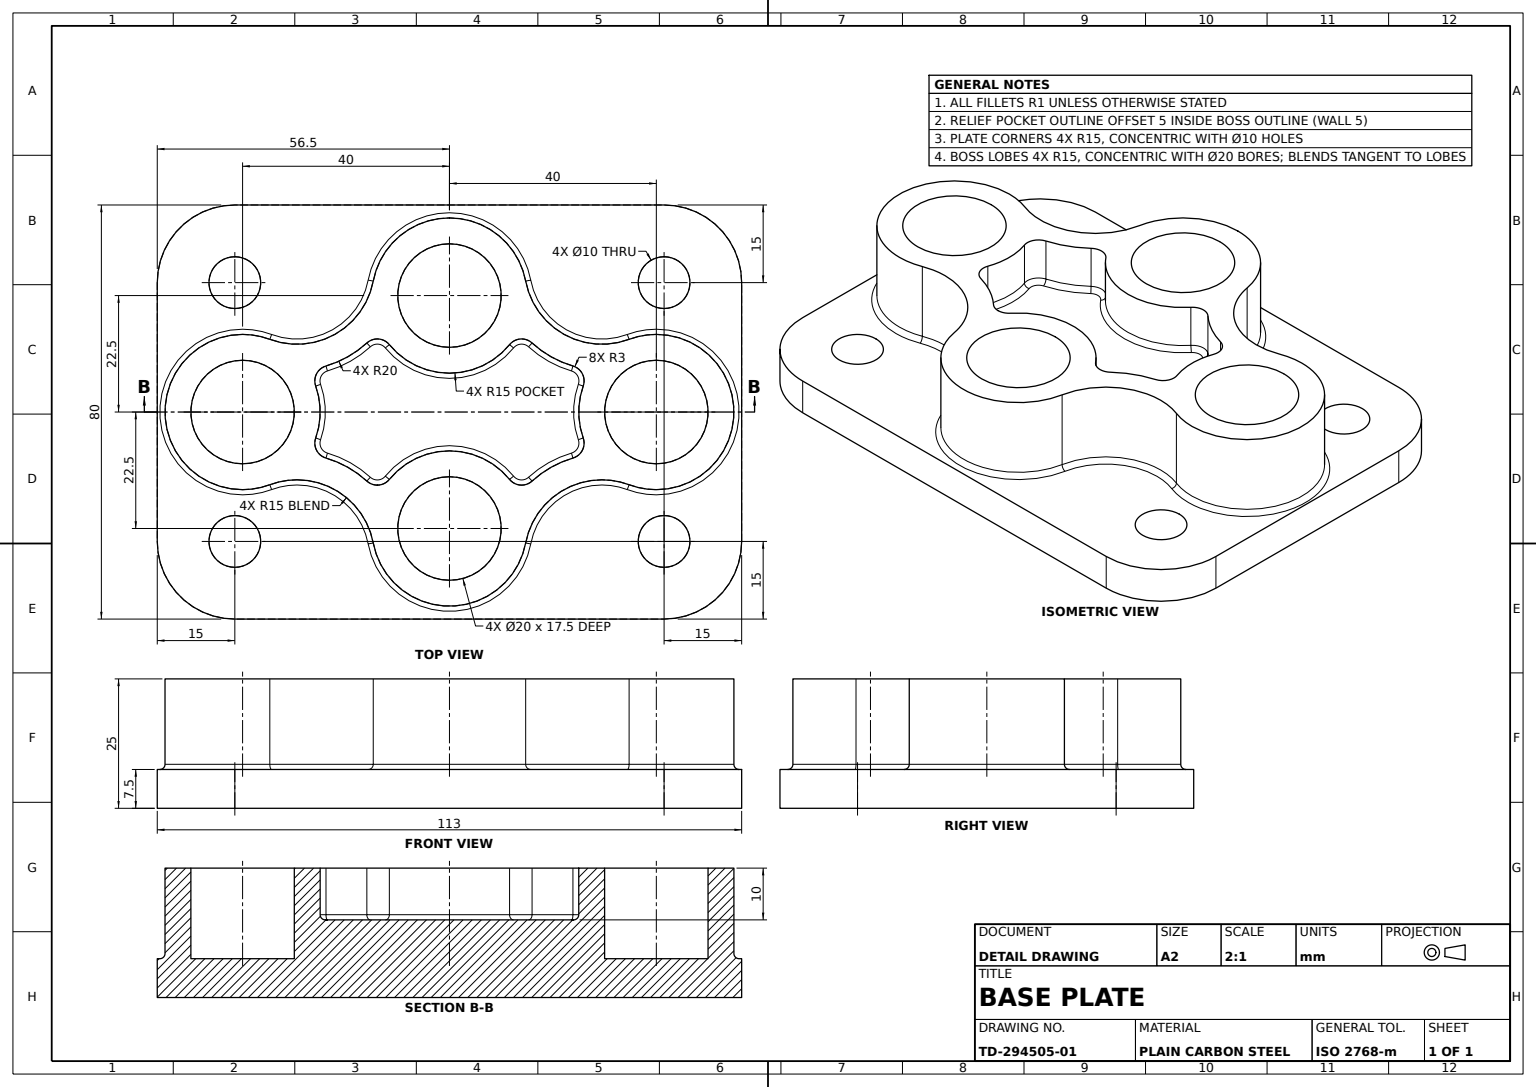
solid
v1 (-56.5,0,25)
v2 (-56.5,7.5,25)
e1 v1 v2 LINE
v3 (-41.5,0,40)
e2 v3 v1 CIRCLE(AX(P(-41.5,0,25),D(0,-1,0),D(0,0,-1)),15)
v4 (-41.5,7.5,40)
e3 v4 v3 LINE
e4 v2 v4 CIRCLE(AX(P(-41.5,7.5,25),D(0,1,0),D(0,0,-1)),15)
face CYL(AX(P(-41.5,7.5,25),D(0,-1,0),D(0,0,-1)),15) [-e1 -e2 -e3 -e4]
v5 (41.5,7.5,20)
v6 (41.5,7.5,30)
e5 v5 v6 CIRCLE(AX(P(41.5,7.5,25),D(0,1,0),D(0,0,1)),5)
v7 (41.5,0,30)
e6 v7 v6 LINE
v8 (41.5,0,20)
e7 v8 v7 CIRCLE(AX(P(41.5,0,25),D(0,1,0),D(0,0,1)),5)
e8 v8 v5 LINE
face CYL(AX(P(41.5,0,25),D(0,1,0),D(0,0,1)),5) rev [e5 -e6 -e7 e8]
v9 (0,7.5,-12.5)
v10 (0,7.5,-32.5)
e9 v9 v10 CIRCLE(AX(P(0,7.5,-22.5),D(0,1,0),D(0,0,1)),10)
e10 v10 v9 CIRCLE(AX(P(0,7.5,-22.5),D(0,1,0),D(0,0,1)),10)
face PLANE(AX(P(0,7.5,0),D(0,-1,0),D(0,0,-1))) rev [e9 e10]
v11 (25.861645,16,5.01068)
v12 (25.861645,25,5.01068)
e11 v11 v12 LINE
v13 (25.861645,25,-5.01068)
e12 v12 v13 CIRCLE(AX(P(40,25,0),D(0,-1,0),D(0,0,1)),15)
v14 (25.861645,16,-5.01068)
e13 v14 v13 LINE
e14 v14 v11 CIRCLE(AX(P(40,16,0),D(0,1,0),D(0,0,1)),15)
face CYL(AX(P(40,15,0),D(0,1,0),D(0,0,1)),15) [e11 e12 -e13 e14]
v15 (40,7.5,-16)
v16 (40,8.5,-15)
e15 v15 v16 CIRCLE(AX(P(40,8.5,-16),D(-1,0,0),D(0,0,1)),1)
v17 (34.38617,7.5,-14.982821)
e16 v17 v15 CIRCLE(AX(P(40,7.5,0),D(0,-1,0),D(0,0,-1)),16)
v18 (34.737034,8.5,-14.046394)
e17 v17 v18 CIRCLE(AX(P(34.38617,8.5,-14.982821),D(-0.936426284,0,0.350864382),D(0.350864382,0,0.936426284)),1)
e18 v16 v18 CIRCLE(AX(P(40,8.5,0),D(0,1,0),D(0,0,-1)),15)
face TORUS(AX(P(40,8.5,0),D(0,-1,0),D(0,0,-1)),16,1) rev [-e15 -e16 e17 -e18]
v19 (40,25,-15)
e19 v19 v16 LINE
v20 (40,25,15)
e20 v20 v19 CIRCLE(AX(P(40,25,0),D(0,1,0),D(0,0,1)),15)
v21 (40,8.5,15)
e21 v20 v21 LINE
e22 v21 v16 CIRCLE(AX(P(40,8.5,0),D(0,1,0),D(0,0,-1)),15)
face CYL(AX(P(40,25,0),D(0,-1,0),D(0,0,-1)),15) [-e19 -e20 e21 e22]
v22 (-12.398933,15,12.387312)
v23 (12.398933,15,12.387312)
e23 v22 v23 CIRCLE(AX(P(0,15,22.5),D(0,-1,0),D(0,0,1)),16)
v24 (-11.624,16,13.019355)
e24 v22 v24 CIRCLE(AX(P(-12.398933,16,12.387312),D(-0.632042977,0,0.774933336),D(0.774933336,0,0.632042977)),1)
v25 (11.624,16,13.019355)
e25 v25 v24 CIRCLE(AX(P(0,16,22.5),D(0,1,0),D(0,0,1)),15)
e26 v23 v25 CIRCLE(AX(P(12.398933,16,12.387312),D(-0.632042977,0,-0.774933336),D(-0.774933336,0,0.632042977)),1)
face TORUS(AX(P(0,16,22.5),D(0,1,0),D(0,0,1)),16,1) rev [-e23 e24 -e25 -e26]
v26 (40,7.5,16)
e27 v26 v21 CIRCLE(AX(P(40,8.5,16),D(1,0,0),D(0,0,-1)),1)
e28 v15 v26 CIRCLE(AX(P(40,7.5,0),D(0,-1,0),D(0,0,-1)),16)
face TORUS(AX(P(40,8.5,0),D(0,-1,0),D(0,0,-1)),16,1) rev [e15 -e22 -e27 -e28]
v27 (-56.5,7.5,-25)
e29 v27 v2 LINE
v28 (-56.5,0,-25)
e30 v27 v28 LINE
e31 v28 v1 LINE
face PLANE(AX(P(-56.5,7.5,40),D(1,0,0),D(0,0,-1))) rev [e1 -e29 e30 e31]
v29 (-13.9488,15,13.123226)
v30 (-13.9488,16,14.123226)
e32 v29 v30 CIRCLE(AX(P(-13.9488,16,13.123226),D(-1,0,0),D(0,0,1)),1)
v31 (-15.298823,15,12.598841)
e33 v31 v29 CIRCLE(AX(P(-13.9488,15,11.123226),D(0,1,0),D(0,0,1)),2)
v32 (-15.973835,16,13.336648)
e34 v32 v31 CIRCLE(AX(P(-15.298823,16,12.598841),D(0.737807048,0,0.675011674),D(0.675011674,0,-0.737807048)),1)
e35 v30 v32 CIRCLE(AX(P(-13.9488,16,11.123226),D(0,-1,0),D(0,0,1)),3)
face TORUS(AX(P(-13.9488,16,11.123226),D(0,1,0),D(0,0,1)),2,1) rev [-e32 -e33 -e34 -e35]
v33 (34.737034,25,-14.046394)
e36 v33 v18 LINE
e37 v19 v33 CIRCLE(AX(P(40,25,0),D(0,1,0),D(0,0,1)),15)
face CYL(AX(P(40,25,0),D(0,-1,0),D(0,0,-1)),15) [-e36 -e37 e19 e18]
v34 (0,25,-32.5)
e38 v34 v10 LINE
v35 (0,25,-12.5)
e39 v34 v35 CIRCLE(AX(P(0,25,-22.5),D(0,1,0),D(0,0,1)),10)
e40 v35 v9 LINE
face CYL(AX(P(0,25,-22.5),D(0,-1,0),D(0,0,-1)),10) rev [-e38 e39 e40 -e10]
v36 (-34.737034,8.5,-14.046394)
v37 (-40,8.5,-15)
e41 v36 v37 CIRCLE(AX(P(-40,8.5,0),D(0,1,0),D(0,0,-1)),15)
v38 (-34.38617,7.5,-14.982821)
e42 v36 v38 CIRCLE(AX(P(-34.38617,8.5,-14.982821),D(0.936426284,0,0.350864382),D(0.350864382,0,-0.936426284)),1)
v39 (-40,7.5,-16)
e43 v39 v38 CIRCLE(AX(P(-40,7.5,0),D(0,-1,0),D(0,0,-1)),16)
e44 v39 v37 CIRCLE(AX(P(-40,8.5,-16),D(-1,0,0),D(0,0,1)),1)
face TORUS(AX(P(-40,8.5,0),D(0,-1,0),D(0,0,-1)),16,1) rev [-e41 e42 -e43 e44]
v40 (-34.737034,25,-14.046394)
e45 v40 v36 LINE
v41 (-14.737034,25,-25.296394)
e46 v41 v40 CIRCLE(AX(P(-29.474069,25,-28.092789),D(0,-1,0),D(0,0,1)),15)
v42 (-14.737034,8.5,-25.296394)
e47 v41 v42 LINE
e48 v42 v36 CIRCLE(AX(P(-29.474069,8.5,-28.092789),D(0,-1,0),D(0,0,-1)),15)
face CYL(AX(P(-29.474069,25,-28.092789),D(0,-1,0),D(0,0,-1)),15) rev [-e45 -e46 e47 e48]
v43 (-11.624,16,-13.019355)
v44 (-11.624,25,-13.019355)
e49 v43 v44 LINE
v45 (0,16,-7.5)
e50 v43 v45 CIRCLE(AX(P(0,16,-22.5),D(0,1,0),D(0,0,1)),15)
v46 (0,25,-7.5)
e51 v45 v46 LINE
e52 v46 v44 CIRCLE(AX(P(0,25,-22.5),D(0,-1,0),D(0,0,1)),15)
face CYL(AX(P(0,15,-22.5),D(0,1,0),D(0,0,1)),15) [-e49 e50 e51 e52]
v47 (23.873986,25,8.892813)
e53 v47 v12 CIRCLE(AX(P(23.033974,25,6.012816),D(0,1,0),D(0,0,1)),3)
v48 (23.873986,16,8.892813)
e54 v11 v48 CIRCLE(AX(P(23.033974,16,6.012816),D(0,-1,0),D(0,0,1)),3)
e55 v48 v47 LINE
face CYL(AX(P(23.033974,15,6.012816),D(0,1,0),D(0,0,1)),3) rev [e53 -e11 e54 e55]
v49 (15.298823,15,12.598841)
v50 (15.973835,16,13.336648)
e56 v49 v50 CIRCLE(AX(P(15.298823,16,12.598841),D(-0.737807048,0,0.675011674),D(0.675011674,0,0.737807048)),1)
v51 (13.9488,15,13.123226)
e57 v51 v49 CIRCLE(AX(P(13.9488,15,11.123226),D(0,1,0),D(0,0,1)),2)
v52 (13.9488,16,14.123226)
e58 v51 v52 CIRCLE(AX(P(13.9488,16,13.123226),D(-1,0,0),D(0,0,1)),1)
e59 v50 v52 CIRCLE(AX(P(13.9488,16,11.123226),D(0,-1,0),D(0,0,1)),3)
face TORUS(AX(P(13.9488,16,11.123226),D(0,1,0),D(0,0,1)),2,1) rev [-e56 -e57 e58 -e59]
v53 (13.9488,25,14.123226)
v54 (15.973835,25,13.336648)
e60 v53 v54 CIRCLE(AX(P(13.9488,25,11.123226),D(0,1,0),D(0,0,-1)),3)
e61 v50 v54 LINE
e62 v52 v53 LINE
face CYL(AX(P(13.9488,15,11.123226),D(0,1,0),D(0,0,1)),3) rev [e60 -e61 e59 e62]
v55 (-15.719503,7.5,-25.482821)
v56 (0,7.5,-38.5)
e63 v55 v56 CIRCLE(AX(P(0,7.5,-22.5),D(0,-1,0),D(0,0,-1)),16)
e64 v42 v55 CIRCLE(AX(P(-15.719503,8.5,-25.482821),D(0.186426284,0,-0.982468951),D(-0.982468951,0,-0.186426284)),1)
v57 (0,8.5,-37.5)
e65 v57 v42 CIRCLE(AX(P(0,8.5,-22.5),D(0,1,0),D(0,0,-1)),15)
e66 v56 v57 CIRCLE(AX(P(0,8.5,-38.5),D(-1,0,0),D(0,0,1)),1)
face TORUS(AX(P(0,8.5,-22.5),D(0,-1,0),D(0,0,-1)),16,1) rev [-e63 -e64 -e65 -e66]
v58 (-41.5,0,-20)
v59 (-41.5,7.5,-20)
e67 v58 v59 LINE
v60 (-41.5,0,-30)
e68 v60 v58 CIRCLE(AX(P(-41.5,0,-25),D(0,1,0),D(0,0,1)),5)
v61 (-41.5,7.5,-30)
e69 v60 v61 LINE
e70 v61 v59 CIRCLE(AX(P(-41.5,7.5,-25),D(0,1,0),D(0,0,1)),5)
face CYL(AX(P(-41.5,0,-25),D(0,1,0),D(0,0,1)),5) rev [-e67 -e68 e69 e70]
v62 (14.737034,8.5,-25.296394)
e71 v18 v62 CIRCLE(AX(P(29.474069,8.5,-28.092789),D(0,-1,0),D(0,0,-1)),15)
v63 (14.737034,25,-25.296394)
e72 v63 v62 LINE
e73 v33 v63 CIRCLE(AX(P(29.474069,25,-28.092789),D(0,-1,0),D(0,0,1)),15)
face CYL(AX(P(29.474069,25,-28.092789),D(0,-1,0),D(0,0,-1)),15) rev [e36 e71 -e72 -e73]
v64 (15.719503,7.5,-25.482821)
e74 v64 v17 CIRCLE(AX(P(29.474069,7.5,-28.092789),D(0,1,0),D(0,0,-1)),14)
e75 v62 v64 CIRCLE(AX(P(15.719503,8.5,-25.482821),D(0.186426284,0,0.982468951),D(0.982468951,0,-0.186426284)),1)
face TORUS(AX(P(29.474069,8.5,-28.092789),D(0,-1,0),D(0,0,-1)),14,1) rev [-e74 -e75 -e71 -e17]
e76 v38 v55 CIRCLE(AX(P(-29.474069,7.5,-28.092789),D(0,1,0),D(0,0,-1)),14)
face TORUS(AX(P(-29.474069,8.5,-28.092789),D(0,-1,0),D(0,0,-1)),14,1) rev [-e48 e64 -e76 -e42]
v65 (-15.719503,7.5,25.482821)
v66 (-29.474069,7.5,14.092789)
e77 v65 v66 CIRCLE(AX(P(-29.474069,7.5,28.092789),D(0,1,0),D(0,0,-1)),14)
v67 (-14.737034,8.5,25.296394)
e78 v65 v67 CIRCLE(AX(P(-15.719503,8.5,25.482821),D(0.186426284,0,0.982468951),D(0.982468951,0,-0.186426284)),1)
v68 (-29.474069,8.5,13.092789)
e79 v68 v67 CIRCLE(AX(P(-29.474069,8.5,28.092789),D(0,-1,0),D(0,0,-1)),15)
e80 v68 v66 CIRCLE(AX(P(-29.474069,8.5,14.092789),D(-1,0,0),D(0,0,1)),1)
face TORUS(AX(P(-29.474069,8.5,28.092789),D(0,-1,0),D(0,0,-1)),14,1) rev [-e77 e78 -e79 e80]
v69 (15.973835,16,-13.336648)
v70 (15.973835,25,-13.336648)
e81 v69 v70 LINE
v71 (23.873986,16,-8.892813)
e82 v69 v71 CIRCLE(AX(P(29.474069,16,-28.092789),D(0,1,0),D(0,0,1)),20)
v72 (23.873986,25,-8.892813)
e83 v71 v72 LINE
e84 v72 v70 CIRCLE(AX(P(29.474069,25,-28.092789),D(0,-1,0),D(0,0,1)),20)
face CYL(AX(P(29.474069,15,-28.092789),D(0,1,0),D(0,0,1)),20) [-e81 e82 e83 e84]
v73 (40,25,-10)
v74 (40,25,10)
e85 v73 v74 CIRCLE(AX(P(40,25,0),D(0,1,0),D(0,0,1)),10)
v75 (40,7.5,10)
e86 v74 v75 LINE
v76 (40,7.5,-10)
e87 v76 v75 CIRCLE(AX(P(40,7.5,0),D(0,1,0),D(0,0,1)),10)
e88 v73 v76 LINE
face CYL(AX(P(40,25,0),D(0,-1,0),D(0,0,-1)),10) rev [e85 e86 -e87 -e88]
v77 (-15.973835,25,13.336648)
e89 v32 v77 LINE
v78 (-23.873986,16,8.892813)
e90 v32 v78 CIRCLE(AX(P(-29.474069,16,28.092789),D(0,1,0),D(0,0,1)),20)
v79 (-23.873986,25,8.892813)
e91 v78 v79 LINE
e92 v79 v77 CIRCLE(AX(P(-29.474069,25,28.092789),D(0,-1,0),D(0,0,1)),20)
face CYL(AX(P(-29.474069,15,28.092789),D(0,1,0),D(0,0,1)),20) [-e89 e90 e91 e92]
e93 v48 v50 CIRCLE(AX(P(29.474069,16,28.092789),D(0,1,0),D(0,0,1)),20)
e94 v54 v47 CIRCLE(AX(P(29.474069,25,28.092789),D(0,-1,0),D(0,0,1)),20)
face CYL(AX(P(29.474069,15,28.092789),D(0,1,0),D(0,0,1)),20) [-e55 e93 e61 e94]
e95 v74 v73 CIRCLE(AX(P(40,25,0),D(0,1,0),D(0,0,1)),10)
e96 v75 v76 CIRCLE(AX(P(40,7.5,0),D(0,1,0),D(0,0,1)),10)
face CYL(AX(P(40,25,0),D(0,-1,0),D(0,0,-1)),10) rev [-e86 e95 e88 -e96]
v80 (34.38617,7.5,14.982821)
v81 (34.737034,8.5,14.046394)
e97 v80 v81 CIRCLE(AX(P(34.38617,8.5,14.982821),D(0.936426284,0,0.350864382),D(0.350864382,0,-0.936426284)),1)
v82 (29.474069,8.5,13.092789)
e98 v82 v81 CIRCLE(AX(P(29.474069,8.5,28.092789),D(0,-1,0),D(0,0,-1)),15)
v83 (29.474069,7.5,14.092789)
e99 v82 v83 CIRCLE(AX(P(29.474069,8.5,14.092789),D(-1,0,0),D(0,0,1)),1)
e100 v80 v83 CIRCLE(AX(P(29.474069,7.5,28.092789),D(0,1,0),D(0,0,-1)),14)
face TORUS(AX(P(29.474069,8.5,28.092789),D(0,-1,0),D(0,0,-1)),14,1) rev [e97 -e98 e99 -e100]
v84 (0,25,12.5)
v85 (0,7.5,12.5)
e101 v84 v85 LINE
v86 (0,7.5,32.5)
e102 v86 v85 CIRCLE(AX(P(0,7.5,22.5),D(0,1,0),D(0,0,1)),10)
v87 (0,25,32.5)
e103 v87 v86 LINE
e104 v87 v84 CIRCLE(AX(P(0,25,22.5),D(0,1,0),D(0,0,1)),10)
face CYL(AX(P(0,25,22.5),D(0,-1,0),D(0,0,-1)),10) rev [e101 -e102 -e103 e104]
v88 (-15.973835,25,-13.336648)
e105 v44 v88 CIRCLE(AX(P(-13.9488,25,-11.123226),D(0,1,0),D(0,0,-1)),3)
v89 (-15.973835,16,-13.336648)
e106 v89 v88 LINE
e107 v89 v43 CIRCLE(AX(P(-13.9488,16,-11.123226),D(0,-1,0),D(0,0,1)),3)
face CYL(AX(P(-13.9488,15,-11.123226),D(0,1,0),D(0,0,1)),3) rev [e49 e105 -e106 e107]
v90 (-15.298823,15,-12.598841)
e108 v89 v90 CIRCLE(AX(P(-15.298823,16,-12.598841),D(-0.737807048,0,0.675011674),D(0.675011674,0,0.737807048)),1)
v91 (-12.398933,15,-12.387312)
e109 v91 v90 CIRCLE(AX(P(-13.9488,15,-11.123226),D(0,1,0),D(0,0,1)),2)
e110 v43 v91 CIRCLE(AX(P(-12.398933,16,-12.387312),D(-0.632042977,0,-0.774933336),D(-0.774933336,0,0.632042977)),1)
face TORUS(AX(P(-13.9488,16,-11.123226),D(0,1,0),D(0,0,1)),2,1) rev [e108 -e109 -e110 -e107]
v92 (41.5,7.5,-40)
v93 (-41.5,7.5,-40)
e111 v92 v93 LINE
v94 (41.5,0,-40)
e112 v92 v94 LINE
v95 (-41.5,0,-40)
e113 v94 v95 LINE
e114 v95 v93 LINE
face PLANE(AX(P(-56.5,7.5,-40),D(0,0,1),D(1,0,0))) rev [-e111 e112 e113 e114]
e115 v6 v5 CIRCLE(AX(P(41.5,7.5,25),D(0,1,0),D(0,0,1)),5)
e116 v7 v8 CIRCLE(AX(P(41.5,0,25),D(0,1,0),D(0,0,1)),5)
face CYL(AX(P(41.5,0,25),D(0,1,0),D(0,0,1)),5) rev [e6 e115 -e8 -e116]
v96 (41.5,0,-20)
v97 (41.5,0,-30)
e117 v96 v97 CIRCLE(AX(P(41.5,0,-25),D(0,1,0),D(0,0,1)),5)
e118 v97 v96 CIRCLE(AX(P(41.5,0,-25),D(0,1,0),D(0,0,1)),5)
v98 (-41.5,0,30)
v99 (-41.5,0,20)
e119 v98 v99 CIRCLE(AX(P(-41.5,0,25),D(0,1,0),D(0,0,1)),5)
e120 v99 v98 CIRCLE(AX(P(-41.5,0,25),D(0,1,0),D(0,0,1)),5)
e121 v58 v60 CIRCLE(AX(P(-41.5,0,-25),D(0,1,0),D(0,0,1)),5)
v100 (41.5,0,40)
e122 v3 v100 LINE
e123 v28 v95 CIRCLE(AX(P(-41.5,0,-25),D(0,-1,0),D(0,0,-1)),15)
v101 (56.5,0,-25)
e124 v94 v101 CIRCLE(AX(P(41.5,0,-25),D(0,-1,0),D(0,0,-1)),15)
v102 (56.5,0,25)
e125 v102 v101 LINE
e126 v102 v100 CIRCLE(AX(P(41.5,0,25),D(0,-1,0),D(0,0,-1)),15)
face PLANE(AX(P(0,0,0),D(0,-1,0),D(0,0,-1))) [e117 e118] [e119 e120] [e68 e121] [e7 e116] [-e122 e2 -e31 e123 -e113 e124 -e125 e126]
v103 (23.593982,15,7.932814)
e127 v103 v48 CIRCLE(AX(P(23.593982,16,7.932814),D(-0.9599988,0,0.280004116),D(0.280004116,0,0.9599988)),1)
v104 (24.919088,15,5.344725)
e128 v104 v11 CIRCLE(AX(P(24.919088,16,5.344725),D(0.334045341,0,0.942557006),D(0.942557006,0,-0.334045341)),1)
e129 v103 v104 CIRCLE(AX(P(23.033974,15,6.012816),D(0,1,0),D(0,0,1)),2)
face TORUS(AX(P(23.033974,16,6.012816),D(0,1,0),D(0,0,1)),2,1) rev [e127 -e54 -e128 -e129]
v105 (-13.9488,25,14.123226)
e130 v77 v105 CIRCLE(AX(P(-13.9488,25,11.123226),D(0,1,0),D(0,0,1)),3)
e131 v30 v105 LINE
face CYL(AX(P(-13.9488,15,11.123226),D(0,1,0),D(0,0,1)),3) rev [e35 e89 e130 -e131]
v106 (15.298823,15,-12.598841)
e132 v106 v69 CIRCLE(AX(P(15.298823,16,-12.598841),D(0.737807048,0,0.675011674),D(0.675011674,0,-0.737807048)),1)
v107 (11.624,16,-13.019355)
e133 v107 v69 CIRCLE(AX(P(13.9488,16,-11.123226),D(0,-1,0),D(0,0,1)),3)
v108 (12.398933,15,-12.387312)
e134 v107 v108 CIRCLE(AX(P(12.398933,16,-12.387312),D(-0.632042977,0,0.774933336),D(0.774933336,0,0.632042977)),1)
e135 v106 v108 CIRCLE(AX(P(13.9488,15,-11.123226),D(0,1,0),D(0,0,1)),2)
face TORUS(AX(P(13.9488,16,-11.123226),D(0,1,0),D(0,0,1)),2,1) rev [e132 -e133 e134 -e135]
v109 (-34.737034,8.5,14.046394)
e136 v109 v68 CIRCLE(AX(P(-29.474069,8.5,28.092789),D(0,-1,0),D(0,0,-1)),15)
v110 (-34.38617,7.5,14.982821)
e137 v109 v110 CIRCLE(AX(P(-34.38617,8.5,14.982821),D(-0.936426284,0,0.350864382),D(0.350864382,0,0.936426284)),1)
e138 v66 v110 CIRCLE(AX(P(-29.474069,7.5,28.092789),D(0,1,0),D(0,0,-1)),14)
face TORUS(AX(P(-29.474069,8.5,28.092789),D(0,-1,0),D(0,0,-1)),14,1) rev [-e80 -e136 e137 -e138]
v111 (-40,7.5,-10)
v112 (-40,7.5,10)
e139 v111 v112 CIRCLE(AX(P(-40,7.5,0),D(0,1,0),D(0,0,1)),10)
e140 v112 v111 CIRCLE(AX(P(-40,7.5,0),D(0,1,0),D(0,0,1)),10)
face PLANE(AX(P(0,7.5,0),D(0,-1,0),D(0,0,-1))) rev [e139 e140]
v113 (-11.624,25,13.019355)
e141 v24 v113 LINE
e142 v24 v30 CIRCLE(AX(P(-13.9488,16,11.123226),D(0,-1,0),D(0,0,1)),3)
e143 v105 v113 CIRCLE(AX(P(-13.9488,25,11.123226),D(0,1,0),D(0,0,1)),3)
face CYL(AX(P(-13.9488,15,11.123226),D(0,1,0),D(0,0,1)),3) rev [-e141 e142 e131 e143]
e144 v13 v72 CIRCLE(AX(P(23.033974,25,-6.012816),D(0,1,0),D(0,0,1)),3)
e145 v71 v14 CIRCLE(AX(P(23.033974,16,-6.012816),D(0,-1,0),D(0,0,1)),3)
face CYL(AX(P(23.033974,15,-6.012816),D(0,1,0),D(0,0,1)),3) rev [e13 e144 -e83 e145]
e146 v59 v61 CIRCLE(AX(P(-41.5,7.5,-25),D(0,1,0),D(0,0,1)),5)
face CYL(AX(P(-41.5,0,-25),D(0,1,0),D(0,0,1)),5) rev [-e121 e67 e146 -e69]
e147 v26 v80 CIRCLE(AX(P(40,7.5,0),D(0,-1,0),D(0,0,-1)),16)
e148 v81 v21 CIRCLE(AX(P(40,8.5,0),D(0,1,0),D(0,0,-1)),15)
face TORUS(AX(P(40,8.5,0),D(0,-1,0),D(0,0,-1)),16,1) rev [-e97 -e147 e27 -e148]
e149 v52 v25 CIRCLE(AX(P(13.9488,16,11.123226),D(0,-1,0),D(0,0,1)),3)
e150 v23 v51 CIRCLE(AX(P(13.9488,15,11.123226),D(0,1,0),D(0,0,1)),2)
face TORUS(AX(P(13.9488,16,11.123226),D(0,1,0),D(0,0,1)),2,1) rev [e26 -e149 -e58 -e150]
e151 v29 v22 CIRCLE(AX(P(-13.9488,15,11.123226),D(0,1,0),D(0,0,1)),2)
face TORUS(AX(P(-13.9488,16,11.123226),D(0,1,0),D(0,0,1)),2,1) rev [-e151 e32 -e142 -e24]
v114 (-41.5,7.5,20)
v115 (-41.5,7.5,30)
e152 v114 v115 CIRCLE(AX(P(-41.5,7.5,25),D(0,1,0),D(0,0,1)),5)
e153 v98 v115 LINE
e154 v99 v114 LINE
face CYL(AX(P(-41.5,0,25),D(0,1,0),D(0,0,1)),5) rev [e152 -e153 -e120 e154]
e155 v56 v64 CIRCLE(AX(P(0,7.5,-22.5),D(0,-1,0),D(0,0,-1)),16)
e156 v62 v57 CIRCLE(AX(P(0,8.5,-22.5),D(0,1,0),D(0,0,-1)),15)
face TORUS(AX(P(0,8.5,-22.5),D(0,-1,0),D(0,0,-1)),16,1) rev [e75 -e155 e66 -e156]
v116 (-23.873986,16,-8.892813)
e157 v116 v89 CIRCLE(AX(P(-29.474069,16,-28.092789),D(0,1,0),D(0,0,1)),20)
v117 (-23.593982,15,-7.932814)
e158 v116 v117 CIRCLE(AX(P(-23.593982,16,-7.932814),D(-0.9599988,0,0.280004116),D(0.280004116,0,0.9599988)),1)
e159 v90 v117 CIRCLE(AX(P(-29.474069,15,-28.092789),D(0,-1,0),D(0,0,1)),21)
face TORUS(AX(P(-29.474069,16,-28.092789),D(0,1,0),D(0,0,1)),21,1) rev [-e157 e158 -e159 -e108]
v118 (41.5,7.5,40)
e160 v100 v118 LINE
e161 v4 v118 LINE
face PLANE(AX(P(-56.5,7.5,40),D(0,0,-1),D(-1,0,0))) rev [e122 e160 -e161 e3]
v119 (0,25,-37.5)
e162 v119 v41 CIRCLE(AX(P(0,25,-22.5),D(0,1,0),D(0,0,1)),15)
e163 v119 v57 LINE
face CYL(AX(P(0,25,-22.5),D(0,-1,0),D(0,0,-1)),15) [-e47 -e162 e163 e65]
v120 (11.624,25,-13.019355)
e164 v70 v120 CIRCLE(AX(P(13.9488,25,-11.123226),D(0,1,0),D(0,0,1)),3)
e165 v107 v120 LINE
face CYL(AX(P(13.9488,15,-11.123226),D(0,1,0),D(0,0,1)),3) rev [e164 -e165 e133 e81]
v121 (-24.919088,15,-5.344725)
v122 (-24.919088,15,5.344725)
e166 v121 v122 CIRCLE(AX(P(-40,15,0),D(0,-1,0),D(0,0,1)),16)
v123 (-25.861645,16,-5.01068)
e167 v123 v121 CIRCLE(AX(P(-24.919088,16,-5.344725),D(0.334045341,0,0.942557006),D(0.942557006,0,-0.334045341)),1)
v124 (-25.861645,16,5.01068)
e168 v124 v123 CIRCLE(AX(P(-40,16,0),D(0,1,0),D(0,0,1)),15)
e169 v124 v122 CIRCLE(AX(P(-24.919088,16,5.344725),D(-0.334045341,0,0.942557006),D(0.942557006,0,0.334045341)),1)
face TORUS(AX(P(-40,16,0),D(0,1,0),D(0,0,1)),16,1) rev [-e166 -e167 -e168 e169]
v125 (41.5,7.5,-30)
e170 v97 v125 LINE
v126 (41.5,7.5,-20)
e171 v96 v126 LINE
e172 v126 v125 CIRCLE(AX(P(41.5,7.5,-25),D(0,1,0),D(0,0,1)),5)
face CYL(AX(P(41.5,0,-25),D(0,1,0),D(0,0,1)),5) rev [-e170 -e117 e171 e172]
e173 v125 v126 CIRCLE(AX(P(41.5,7.5,-25),D(0,1,0),D(0,0,1)),5)
face CYL(AX(P(41.5,0,-25),D(0,1,0),D(0,0,1)),5) rev [-e171 -e118 e170 e173]
e174 v35 v34 CIRCLE(AX(P(0,25,-22.5),D(0,1,0),D(0,0,1)),10)
face CYL(AX(P(0,25,-22.5),D(0,-1,0),D(0,0,-1)),10) rev [-e40 e174 e38 -e9]
e175 v84 v87 CIRCLE(AX(P(0,25,22.5),D(0,1,0),D(0,0,1)),10)
v127 (-25.861645,25,5.01068)
e176 v127 v79 CIRCLE(AX(P(-23.033974,25,6.012816),D(0,1,0),D(0,0,-1)),3)
v128 (-25.861645,25,-5.01068)
e177 v128 v127 CIRCLE(AX(P(-40,25,0),D(0,-1,0),D(0,0,1)),15)
v129 (-23.873986,25,-8.892813)
e178 v129 v128 CIRCLE(AX(P(-23.033974,25,-6.012816),D(0,1,0),D(0,0,-1)),3)
e179 v88 v129 CIRCLE(AX(P(-29.474069,25,-28.092789),D(0,-1,0),D(0,0,1)),20)
e180 v120 v46 CIRCLE(AX(P(0,25,-22.5),D(0,-1,0),D(0,0,1)),15)
v130 (11.624,25,13.019355)
e181 v130 v53 CIRCLE(AX(P(13.9488,25,11.123226),D(0,1,0),D(0,0,-1)),3)
e182 v113 v130 CIRCLE(AX(P(0,25,22.5),D(0,-1,0),D(0,0,1)),15)
v131 (-40,25,-10)
v132 (-40,25,10)
e183 v131 v132 CIRCLE(AX(P(-40,25,0),D(0,1,0),D(0,0,1)),10)
e184 v132 v131 CIRCLE(AX(P(-40,25,0),D(0,1,0),D(0,0,1)),10)
e185 v63 v119 CIRCLE(AX(P(0,25,-22.5),D(0,1,0),D(0,0,1)),15)
v133 (-40,25,-15)
e186 v40 v133 CIRCLE(AX(P(-40,25,0),D(0,1,0),D(0,0,1)),15)
v134 (-40,25,15)
e187 v133 v134 CIRCLE(AX(P(-40,25,0),D(0,1,0),D(0,0,1)),15)
v135 (-34.737034,25,14.046394)
e188 v134 v135 CIRCLE(AX(P(-40,25,0),D(0,1,0),D(0,0,1)),15)
v136 (-29.474069,25,13.092789)
e189 v135 v136 CIRCLE(AX(P(-29.474069,25,28.092789),D(0,-1,0),D(0,0,-1)),15)
v137 (-14.737034,25,25.296394)
e190 v136 v137 CIRCLE(AX(P(-29.474069,25,28.092789),D(0,-1,0),D(0,0,-1)),15)
v138 (14.737034,25,25.296394)
e191 v137 v138 CIRCLE(AX(P(0,25,22.5),D(0,1,0),D(0,0,1)),15)
v139 (29.474069,25,13.092789)
e192 v138 v139 CIRCLE(AX(P(29.474069,25,28.092789),D(0,-1,0),D(0,0,-1)),15)
v140 (34.737034,25,14.046394)
e193 v139 v140 CIRCLE(AX(P(29.474069,25,28.092789),D(0,-1,0),D(0,0,-1)),15)
e194 v140 v20 CIRCLE(AX(P(40,25,0),D(0,1,0),D(0,0,1)),15)
face PLANE(AX(P(-14.737034,25,-25.296394),D(0,1,0),D(0,0,1))) [-e85 -e95] [-e175 -e104] [-e92 -e176 -e177 -e178 -e179 -e105 -e52 -e180 -e164 -e84 -e144 -e12 -e53 -e94 -e60 -e181 -e182 -e143 -e130] [-e39 -e174] [-e183 -e184] [e37 e73 e185 e162 e46 e186 e187 e188 e189 e190 e191 e192 e193 e194 e20]
e195 v124 v127 LINE
e196 v123 v128 LINE
face CYL(AX(P(-40,15,0),D(0,1,0),D(0,0,1)),15) [-e195 e168 e196 e177]
e197 v117 v121 CIRCLE(AX(P(-23.033974,15,-6.012816),D(0,1,0),D(0,0,1)),2)
v141 (-23.593982,15,7.932814)
e198 v122 v141 CIRCLE(AX(P(-23.033974,15,6.012816),D(0,1,0),D(0,0,1)),2)
e199 v141 v31 CIRCLE(AX(P(-29.474069,15,28.092789),D(0,-1,0),D(0,0,1)),21)
e200 v49 v103 CIRCLE(AX(P(29.474069,15,28.092789),D(0,-1,0),D(0,0,1)),21)
v142 (24.919088,15,-5.344725)
e201 v104 v142 CIRCLE(AX(P(40,15,0),D(0,-1,0),D(0,0,1)),16)
v143 (23.593982,15,-7.932814)
e202 v142 v143 CIRCLE(AX(P(23.033974,15,-6.012816),D(0,1,0),D(0,0,1)),2)
e203 v143 v106 CIRCLE(AX(P(29.474069,15,-28.092789),D(0,-1,0),D(0,0,1)),21)
v144 (0,15,-6.5)
e204 v108 v144 CIRCLE(AX(P(0,15,-22.5),D(0,-1,0),D(0,0,1)),16)
e205 v144 v91 CIRCLE(AX(P(0,15,-22.5),D(0,-1,0),D(0,0,1)),16)
face PLANE(AX(P(-26.254021,15,17.052802),D(0,1,0),D(0,0,1))) [e197 e166 e198 e199 e33 e151 e23 e150 e57 e200 e129 e201 e202 e203 e135 e204 e205 e109 e159]
v145 (-40,7.5,16)
v146 (-40,8.5,15)
e206 v145 v146 CIRCLE(AX(P(-40,8.5,16),D(1,0,0),D(0,0,-1)),1)
e207 v110 v145 CIRCLE(AX(P(-40,7.5,0),D(0,-1,0),D(0,0,-1)),16)
e208 v146 v109 CIRCLE(AX(P(-40,8.5,0),D(0,1,0),D(0,0,-1)),15)
face TORUS(AX(P(-40,8.5,0),D(0,-1,0),D(0,0,-1)),16,1) rev [-e206 -e207 -e137 -e208]
e209 v143 v71 CIRCLE(AX(P(23.593982,16,-7.932814),D(0.9599988,0,0.280004116),D(0.280004116,0,-0.9599988)),1)
face TORUS(AX(P(29.474069,16,-28.092789),D(0,1,0),D(0,0,1)),21,1) rev [-e82 -e132 -e203 e209]
e210 v139 v82 LINE
e211 v140 v81 LINE
face CYL(AX(P(29.474069,25,28.092789),D(0,-1,0),D(0,0,-1)),15) rev [-e193 e210 e98 -e211]
e212 v142 v14 CIRCLE(AX(P(24.919088,16,-5.344725),D(-0.334045341,0,0.942557006),D(0.942557006,0,0.334045341)),1)
face TORUS(AX(P(40,16,0),D(0,1,0),D(0,0,1)),16,1) rev [-e201 e128 -e14 -e212]
e213 v123 v116 CIRCLE(AX(P(-23.033974,16,-6.012816),D(0,-1,0),D(0,0,1)),3)
e214 v116 v129 LINE
face CYL(AX(P(-23.033974,15,-6.012816),D(0,1,0),D(0,0,1)),3) rev [e213 e214 e178 -e196]
e215 v132 v112 LINE
e216 v131 v111 LINE
face CYL(AX(P(-40,25,0),D(0,-1,0),D(0,0,-1)),10) rev [-e215 e184 e216 -e140]
e217 v137 v67 LINE
e218 v136 v68 LINE
face CYL(AX(P(-29.474069,25,28.092789),D(0,-1,0),D(0,0,-1)),15) rev [-e217 -e190 e218 e79]
face CYL(AX(P(40,25,0),D(0,-1,0),D(0,0,-1)),15) [-e21 -e194 e211 e148]
e219 v85 v86 CIRCLE(AX(P(0,7.5,22.5),D(0,1,0),D(0,0,1)),10)
face PLANE(AX(P(0,7.5,0),D(0,-1,0),D(0,0,-1))) rev [e219 e102]
e220 v93 v27 CIRCLE(AX(P(-41.5,7.5,-25),D(0,1,0),D(0,0,-1)),15)
face CYL(AX(P(-41.5,7.5,-25),D(0,-1,0),D(0,0,-1)),15) [-e220 -e114 -e123 -e30]
face CYL(AX(P(-40,25,0),D(0,-1,0),D(0,0,-1)),10) rev [e215 -e139 -e216 e183]
e221 v134 v146 LINE
e222 v133 v37 LINE
e223 v37 v146 CIRCLE(AX(P(-40,8.5,0),D(0,1,0),D(0,0,-1)),15)
face CYL(AX(P(-40,25,0),D(0,-1,0),D(0,0,-1)),15) [-e221 -e187 e222 e223]
e224 v78 v124 CIRCLE(AX(P(-23.033974,16,6.012816),D(0,-1,0),D(0,0,1)),3)
face CYL(AX(P(-23.033974,15,6.012816),D(0,1,0),D(0,0,1)),3) rev [e195 e176 -e91 e224]
e225 v78 v141 CIRCLE(AX(P(-23.593982,16,7.932814),D(0.9599988,0,0.280004116),D(0.280004116,0,-0.9599988)),1)
face TORUS(AX(P(-23.033974,16,6.012816),D(0,1,0),D(0,0,1)),2,1) rev [-e169 -e224 e225 -e198]
face TORUS(AX(P(-29.474069,16,28.092789),D(0,1,0),D(0,0,1)),21,1) rev [-e199 -e225 -e90 e34]
e226 v45 v107 CIRCLE(AX(P(0,16,-22.5),D(0,1,0),D(0,0,1)),15)
e227 v45 v144 CIRCLE(AX(P(0,16,-6.5),D(-1,0,0),D(0,0,1)),1)
face TORUS(AX(P(0,16,-22.5),D(0,1,0),D(0,0,1)),16,1) rev [-e134 -e226 e227 -e204]
e228 v145 v39 CIRCLE(AX(P(-40,7.5,0),D(0,-1,0),D(0,0,-1)),16)
face TORUS(AX(P(-40,8.5,0),D(0,-1,0),D(0,0,-1)),16,1) rev [-e44 -e228 e206 -e223]
v147 (15.719503,7.5,25.482821)
e229 v83 v147 CIRCLE(AX(P(29.474069,7.5,28.092789),D(0,1,0),D(0,0,-1)),14)
v148 (14.737034,8.5,25.296394)
e230 v148 v82 CIRCLE(AX(P(29.474069,8.5,28.092789),D(0,-1,0),D(0,0,-1)),15)
e231 v147 v148 CIRCLE(AX(P(15.719503,8.5,25.482821),D(0.186426284,0,-0.982468951),D(-0.982468951,0,-0.186426284)),1)
face TORUS(AX(P(29.474069,8.5,28.092789),D(0,-1,0),D(0,0,-1)),14,1) rev [-e229 -e99 -e230 -e231]
v149 (56.5,7.5,25)
e232 v149 v102 LINE
e233 v118 v149 CIRCLE(AX(P(41.5,7.5,25),D(0,1,0),D(0,0,-1)),15)
face CYL(AX(P(41.5,7.5,25),D(0,-1,0),D(0,0,-1)),15) [-e126 -e232 -e233 -e160]
v150 (56.5,7.5,-25)
e234 v101 v150 LINE
e235 v150 v92 CIRCLE(AX(P(41.5,7.5,-25),D(0,1,0),D(0,0,-1)),15)
face CYL(AX(P(41.5,7.5,-25),D(0,-1,0),D(0,0,-1)),15) [-e234 -e124 -e112 -e235]
face TORUS(AX(P(0,16,-22.5),D(0,1,0),D(0,0,1)),16,1) rev [-e50 e110 -e205 -e227]
e236 v115 v114 CIRCLE(AX(P(-41.5,7.5,25),D(0,1,0),D(0,0,1)),5)
face CYL(AX(P(-41.5,0,25),D(0,1,0),D(0,0,1)),5) rev [-e119 e153 e236 -e154]
face CYL(AX(P(0,15,-22.5),D(0,1,0),D(0,0,1)),15) [-e51 e226 e165 e180]
e237 v147 v65 CIRCLE(AX(P(0,7.5,22.5),D(0,-1,0),D(0,0,-1)),16)
e238 v149 v150 LINE
face PLANE(AX(P(0,7.5,0),D(0,-1,0),D(0,0,-1))) rev [-e173 -e172] [e147 e100 e229 e237 e77 e138 e207 e228 e43 e76 e63 e155 e74 e16 e28] [e233 e238 e235 e111 e220 e29 e4 e161] [-e115 -e5] [-e152 -e236] [-e146 -e70]
face CYL(AX(P(-29.474069,15,-28.092789),D(0,1,0),D(0,0,1)),20) [-e214 e157 e106 e179]
e239 v135 v109 LINE
face CYL(AX(P(-40,25,0),D(0,-1,0),D(0,0,-1)),15) [e221 e208 -e239 -e188]
face CYL(AX(P(0,25,-22.5),D(0,-1,0),D(0,0,-1)),15) [e72 e156 -e163 -e185]
face PLANE(AX(P(56.5,7.5,40),D(-1,0,0),D(0,0,1))) rev [e125 e234 -e238 e232]
face TORUS(AX(P(23.033974,16,-6.012816),D(0,1,0),D(0,0,1)),2,1) rev [-e209 -e202 e212 -e145]
face CYL(AX(P(-29.474069,25,28.092789),D(0,-1,0),D(0,0,-1)),15) rev [-e218 -e189 e239 e136]
face CYL(AX(P(0,25,22.5),D(0,-1,0),D(0,0,-1)),10) rev [e103 -e219 -e101 e175]
e240 v138 v148 LINE
face CYL(AX(P(29.474069,25,28.092789),D(0,-1,0),D(0,0,-1)),15) rev [-e210 -e192 e240 e230]
face TORUS(AX(P(29.474069,16,28.092789),D(0,1,0),D(0,0,1)),21,1) rev [-e127 -e200 e56 -e93]
face CYL(AX(P(-40,25,0),D(0,-1,0),D(0,0,-1)),15) [e41 -e222 -e186 e45]
e241 v67 v148 CIRCLE(AX(P(0,8.5,22.5),D(0,1,0),D(0,0,-1)),15)
face CYL(AX(P(0,25,22.5),D(0,-1,0),D(0,0,-1)),15) [e217 e241 -e240 -e191]
e242 v25 v130 LINE
face CYL(AX(P(13.9488,15,11.123226),D(0,1,0),D(0,0,1)),3) rev [e149 e242 e181 -e62]
face TORUS(AX(P(-23.033974,16,-6.012816),D(0,1,0),D(0,0,1)),2,1) rev [-e197 -e158 -e213 e167]
face CYL(AX(P(0,15,22.5),D(0,1,0),D(0,0,1)),15) [e25 e141 e182 -e242]
face PLANE(AX(P(0,7.5,0),D(0,-1,0),D(0,0,-1))) rev [e96 e87]
face TORUS(AX(P(0,8.5,22.5),D(0,-1,0),D(0,0,-1)),16,1) rev [e231 -e241 -e78 -e237]
